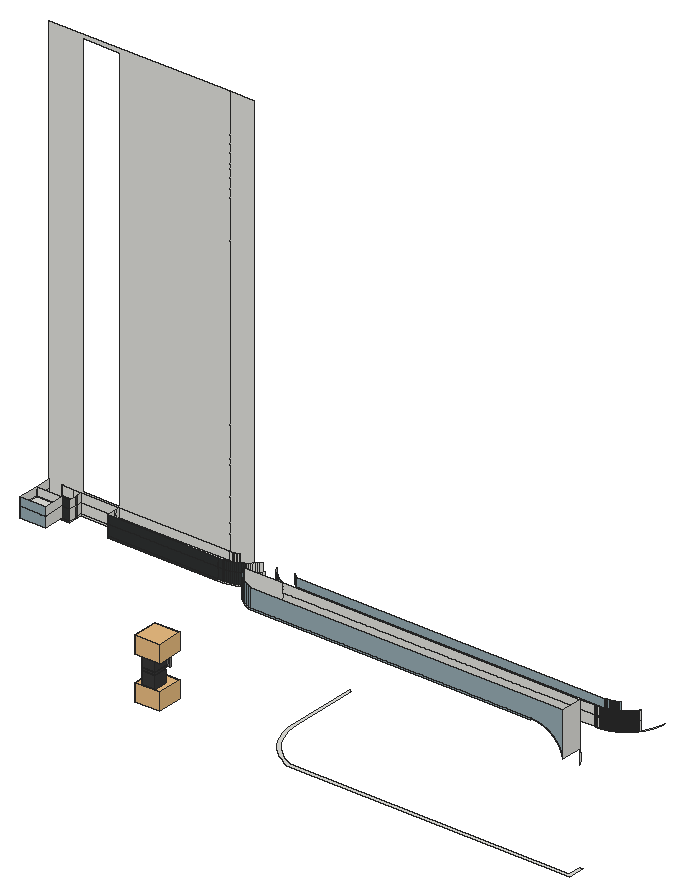
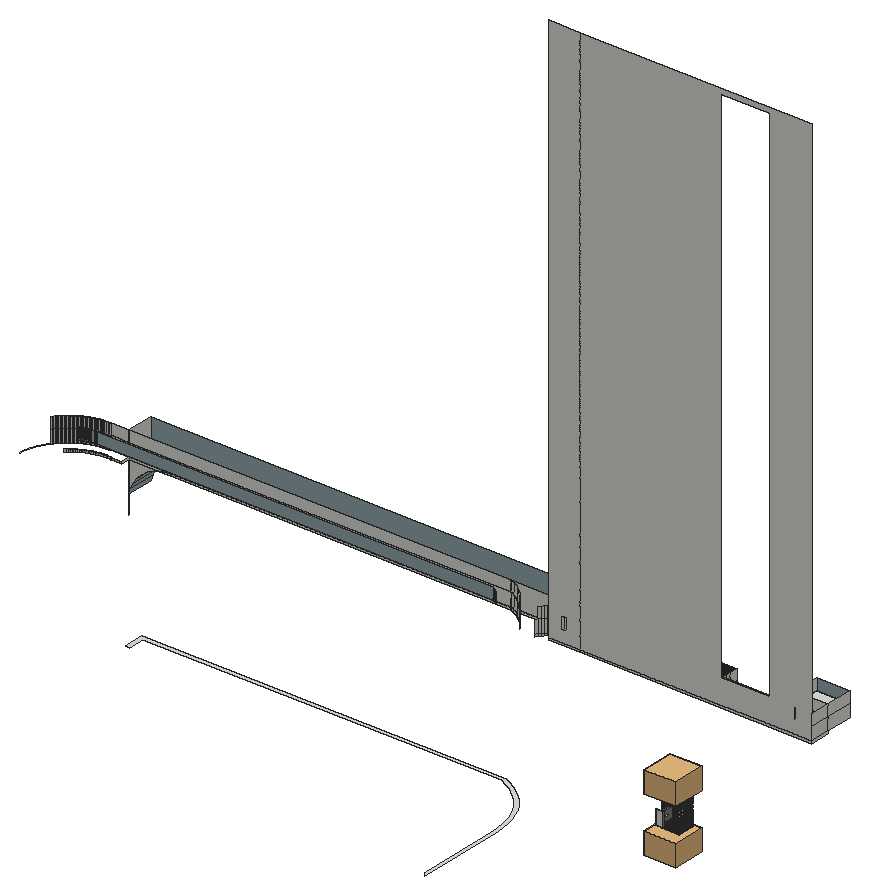
# SketchUp Ruby script. Lengths in inches.
U = 1.inch
M = Sketchup.active_model
def pt(a) = Geom::Point3d.new(a.map { |v| v * U })
def face(e, loops, mat)
  f = e.add_face(loops[0].map { |a| pt(a) })
  loops[1..].each { |l| e.add_face(l.map { |a| pt(a) }).erase! }
  f.material = f.back_material = mat if mat
  f
end
# faces: each face lists its corners as indices into pts; further lists are holes
def faces(e, pts, list, mat = nil) = list.each { |f| face(e, (f[0].is_a?(Array) ? f : [f]).map { |l| l.map { |i| pts[i] } }, mat) }
# xy, xz, yz: faces in a plane at the given z, y or x. An outline is a flat list of corners, or four numbers for a rectangle; further outlines are holes
def ring(l) = l.size == 4 ? [[l[0], l[1]], [l[2], l[1]], [l[2], l[3]], [l[0], l[3]]] : l.each_slice(2).to_a
def flat(e, list, mat, &to3) = list.each { |f| face(e, (f[0].is_a?(Array) ? f : [f]).map { |l| ring(l).map { |u, v| to3.(u, v) } }, mat) }
def xy(e, z, list, mat = nil) = flat(e, list, mat) { |x, y| [x, y, z] }
def xz(e, y, list, mat = nil) = flat(e, list, mat) { |x, z| [x, y, z] }
def yz(e, x, list, mat = nil) = flat(e, list, mat) { |y, z| [x, y, z] }
def lines(e, pts, list) = list.each { |a, b| e.add_line(pt(pts[a]), pt(pts[b])) }
# prism: a flat outline (further loops are holes) pulled along v
def prism(e, loops, v, mat = nil)
  f = face(e, loops, mat); d = Geom::Vector3d.new(v.map { |x| x * U })
  f.pushpull(f.normal.samedirection?(d) ? d.length : -d.length)
end
def box(e, o, s, mat = nil) = prism(e, [[o, [o[0] + s[0], o[1], o[2]], [o[0] + s[0], o[1] + s[1], o[2]], [o[0], o[1] + s[1], o[2]]]], [0, 0, s[2]], mat)
def at(x, y, z, deg = 0) = Geom::Transformation.translation(pt([x, y, z])) * Geom::Transformation.rotation(ORIGIN, Z_AXIS, deg.degrees)
def axes(o, x, y, z) = Geom::Transformation.new([*x, 0, *y, 0, *z, 0, *pt(o).to_a, 1])
def part(name) = M.definitions.add(name)
# library, detail: a bought-in or finely detailed component or shape, given as its bounding box
def library(name, o, s) = part(name).tap { |d| box(d.entities, o, s) }
def detail(e, o, s) = box(e.add_group.entities, o, s)
def put(e, d, t, mat = nil) = e.add_instance(d, t).tap { |i| i.material = mat if mat }
def group(e, t, mat = nil) = e.add_group.tap { |g| g.transformation = t; g.material = mat if mat }.entities
root = M.entities
M.materials.add("11.free-metal-textures").color = [58, 58, 58]
M.materials.add("Generic").color = [150, 171, 178]
M.materials.add("Generic\#1").color = [47, 50, 50]
M.materials.add("Glass Thin Clear 001").color = [252, 250, 250]
M.materials["Glass Thin Clear 001"].alpha = 0.1
M.materials.add("[0111_SlateGray]").color = [112, 128, 144]
M.materials.add("[0117_GhostWhite]").color = [248, 248, 255]
M.materials.add("images").color = [124, 124, 124]
c1 = library("Spot Light",[-7.3,-7.3,-9.9375],[14.6,14.6,9.9375])
c2 = part("Group0\#1")
p = [[-17.97,0.98,0],[-6.48,-16.79,0],[0,0,38],[13.97,-11.35,0],[15.11,9.78,0],[-4.625,17.4,0]]
faces(c2.entities,p,[[0,1,2],[1,3,2],[3,4,2],[5,0,2],[4,5,2]])
c3 = part("wall light")
g1 = group(c3.entities,at(188.14,62.59,-1.03))
xy(g1,0.24,[[[0,0,7.875,7.875],[0.49,0.49,7.38,7.38]]],"images")
xy(g1,1.03,[[[0.49,0.49,7.38,7.38],[0.73,0.73,7.14,7.14]]],"[0111_SlateGray]")
xy(g1,2.21,[[0.73,0.73,7.14,7.14]],"[0117_GhostWhite]")
xy(g1,5.75,[[2.36,13.78,5.51,14.17]],"images")
xy(g1,6.74,[[3.35,7.875,4.52,13.78]],"images")
xy(g1,7.72,[[0,0,7.875,0,7.875,7.875,7.38,7.875,7.38,0.49,0.49,0.49,0.49,7.875,0,7.875],[0.49,7.38,7.38,7.875]])
xy(g1,8.5,[[3.35,9.63,4.52,12.02]])
xy(g1,8.51,[[0,0,0,7.875,0.49,7.875,0.49,0.49,7.38,0.49,7.38,7.875,7.875,7.875,7.875,0]])
xy(g1,9.29,[[0,0,7.875,0,7.875,7.875,7.38,7.875,7.38,0.49,0.49,0.49,0.49,7.875,0,7.875]])
xy(g1,9.3,[[3.35,9.63,4.52,12.02]])
xy(g1,10.08,[[0,0,7.875,0,7.875,7.875,7.38,7.875,7.38,0.49,0,0.49],[0,0.49,0.49,7.875],[0.49,7.38,7.38,7.875]])
xy(g1,11.06,[[3.35,7.875,4.52,13.78]],"images")
xy(g1,12.05,[[2.36,13.78,5.51,14.17]],"images")
xy(g1,15.59,[[0.73,0.73,7.14,7.14]],"[0117_GhostWhite]")
xy(g1,16.77,[[[0.49,0.49,7.38,7.38],[0.73,0.73,7.14,7.14]]],"[0111_SlateGray]")
xy(g1,17.5625,[[[0,0,7.875,7.875],[0.49,0.49,7.38,7.38]]],"images")
xz(g1,0,[[0,0.24,7.875,7.72],[0,8.51,7.875,9.29],[0,10.08,7.875,17.5625]],"11.free-metal-textures")
xz(g1,0.49,[[0.49,8.51,7.38,8.9],[0.49,8.9,7.38,9.29]])
xz(g1,0.49,[[0.49,0.24,7.38,1.03],[0.49,16.77,7.38,17.5625]],"[0111_SlateGray]")
xz(g1,0.49,[[0.49,7.72,7.38,8.51],[0.49,9.29,7.38,10.08]],"[0117_GhostWhite]")
xz(g1,0.73,[[0.73,1.03,7.14,2.21],[0.73,2.21,7.14,15.59],[0.73,15.59,7.14,16.77]],"[0111_SlateGray]")
xz(g1,7.14,[[0.73,1.03,7.14,2.21],[0.73,2.21,7.14,15.59],[0.73,15.59,7.14,16.77]],"[0111_SlateGray]")
xz(g1,7.38,[[0.49,0.24,7.38,1.03],[0.49,16.77,7.38,17.5625]],"[0111_SlateGray]")
xz(g1,7.875,[[3.35,6.74,4.52,7.72],[3.35,7.72,3.9375,10.08],[3.9375,7.72,4.52,10.08],[3.35,10.08,4.52,11.06]])
xz(g1,7.875,[[0,0.24,0,7.72,3.35,7.72,3.35,6.74,4.52,6.74,4.52,7.72,7.875,7.72,7.875,0.24],[0.49,7.72,0.49,8.51,0,8.51,0,9.29,0.49,9.29,0.49,10.08,3.35,10.08,3.35,7.72],[4.52,7.72,4.52,10.08,7.38,10.08,7.38,9.29,7.875,9.29,7.875,8.51,7.38,8.51,7.38,7.72],[0,10.08,0,17.5625,7.875,17.5625,7.875,10.08,4.52,10.08,4.52,11.06,3.35,11.06,3.35,10.08]],"11.free-metal-textures")
xz(g1,9.63,[[3.35,8.5,4.52,9.3]])
xz(g1,12.02,[[3.35,8.5,4.52,9.3]])
xz(g1,13.78,[[2.36,5.75,4.52,5.75,4.52,6.74,3.35,6.74,3.35,11.06,4.52,11.06,4.52,5.75,5.51,5.75,5.51,12.05,2.36,12.05]],"images")
xz(g1,14.17,[[2.36,5.75,5.51,12.05]])
yz(g1,0,[[0,0.24,7.875,7.72],[0,8.51,7.875,9.29],[0,10.08,7.875,17.5625]],"11.free-metal-textures")
yz(g1,0.49,[[0.49,8.51,7.38,8.9]])
yz(g1,0.49,[[0.49,0.24,7.38,1.03],[0.49,16.77,7.38,17.5625]],"[0111_SlateGray]")
yz(g1,0.49,[[0.49,7.72,7.875,8.51],[0.49,9.29,7.875,10.08]],"[0117_GhostWhite]")
yz(g1,0.73,[[0.73,1.03,7.14,2.21],[0.73,2.21,7.14,15.59],[0.73,15.59,7.14,16.77]],"[0111_SlateGray]")
yz(g1,2.36,[[13.78,5.75,14.17,12.05]],"images")
yz(g1,3.35,[[[7.875,6.74,13.78,11.06],[9.63,8.5,12.02,9.3]]],"images")
yz(g1,4.52,[[[7.875,6.74,13.78,11.06],[9.63,8.5,12.02,9.3]]],"images")
yz(g1,5.51,[[13.78,5.75,14.17,12.05]],"images")
yz(g1,7.14,[[0.73,1.03,7.14,2.21],[0.73,2.21,7.14,15.59],[0.73,15.59,7.14,16.77]],"[0111_SlateGray]")
yz(g1,7.38,[[0.49,8.51,7.38,8.9]])
yz(g1,7.38,[[0.49,0.24,7.38,1.03],[0.49,16.77,7.38,17.5625]],"[0111_SlateGray]")
yz(g1,7.38,[[0.49,7.72,7.875,8.51],[0.49,9.29,7.875,10.08]],"[0117_GhostWhite]")
yz(g1,7.875,[[0,0.24,7.875,7.72],[0,8.51,7.875,9.29],[0,10.08,7.875,17.5625]],"11.free-metal-textures")
p = [[7.38,7.38,8.9],[0.49,7.38,8.9],[4.52,7.875,6.54],[4.52,7.875,6.74],[4.52,13.78,5.5625],[4.52,13.78,5.75]]
lines(g1,p,[[0,1],[2,3],[4,5]])
put(g1,c2,axes([3.74,4.28,0],[0.1617,0,0],[0,0.1617,0],[0,0,0.1617]))
put(g1,c2,axes([4.15,3.625,18],[-0.1617,0,0],[0,0.1617,0],[0,0,-0.1617]))
xy(root,168.5625,[[164.303,33.128,330.023,33.128,330.023,42.441,328.27,42.441,328.27,34.881,164.664,34.881,162.347,35.879,159.469,37.48,156.769,39.364,154.272,41.512,152.005,43.9,149.992,46.506,148.252,49.301,146.803,52.258,145.661,55.347,144.836,58.535,144.338,61.79,144.165,65.204,144.165,104.598,142.412,106.351,142.412,65.159,142.591,61.612,143.116,58.182,143.985,54.822,145.189,51.567,146.716,48.45,148.55,45.504,150.673,42.758,153.062,40.24,155.693,37.977,158.539,35.992,161.572,34.304]])
xy(root,245,[[145.638,29.933,143.73,30.488,141.889,31.231,140.131,32.157,138.476,33.255,136.939,34.513,135.537,35.921,134.284,37.462,133.193,39.122,132.274,40.883,131.803,42.0625,309.912,42.0625,309.912,29.933]],"Generic")
xy(root,246,[[10.218,29.933,25.218,42.0625],[145.638,29.933,309.912,29.933,309.912,42.0625,131.803,42.0625,132.274,40.883,133.193,39.122,134.284,37.462,135.537,35.921,136.939,34.513,138.476,33.255,140.131,32.157,141.889,31.231,143.73,30.488],[119.415,42.0625,120.438,42.148,121.455,42.289,122.463,42.485,123.459,42.737,124.439,43.042,125.401,43.4,126.342,43.81,127.26,44.271,128.151,44.781,129.013,45.339,129.843,45.943,130.639,46.592,129.741,45.931,128.812,45.317,127.853,44.749,126.867,44.231,125.856,43.763,124.822,43.346,123.769,42.981,122.699,42.67,121.615,42.412,120.52,42.21],[131.803,42.0625,131.651,42.423,131.509,42.788,131.377,43.156,131.254,43.528,131.142,43.903,131.039,44.28,130.947,44.661,130.865,45.043,130.793,45.428,130.731,45.814,130.68,46.202,130.639,46.592,130.991,44.637,131.538,42.727],[337.222,42.0625,337.846,42.071,338.474,42.095,339.101,42.136,339.638,42.186],
  [339.638,42.186,339.726,42.194,340.35,42.268,340.972,42.358,341.591,42.464,342.207,42.587,342.82,42.726,343.429,42.88,344.034,43.051,344.634,43.237,345.229,43.439,345.818,43.657,346.402,43.889,346.979,44.137,347.55,44.4,348.113,44.678,348.669,44.971,349.218,45.278,349.758,45.599,350.289,45.934,350.811,46.283,351.324,46.646,351.828,47.022,352.321,47.411,352.804,47.813,353.277,48.227,353.738,48.654,354.188,49.092,354.627,49.542,355.053,50.003,355.467,50.476,355.869,50.959,356.258,51.452,356.634,51.956,356.997,52.469,357.346,52.991,357.681,53.523,358.002,54.0625,358.309,54.611,358.602,55.167,358.88,55.73,359.143,56.301,359.391,56.878,359.624,57.462,359.841,58.051,360.043,58.646,360.229,59.246,360.4,59.851,360.554,60.46,360.693,61.073,360.816,61.689,360.922,62.308,361.012,62.93,361.086,63.554,361.094,63.642,361.086,63.17,361.031,62.701,360.967,62.234,360.893,61.768,360.81,61.304,360.718,60.841,360.617,60.381,360.506,59.922,360.387,59.466,360.258,59.012,360.12,58.561,359.973,58.113,359.818,57.668,359.653,57.226,359.48,56.787,359.298,56.352,359.107,55.921,358.908,55.494,358.701,55.07,358.484,54.651,358.26,54.236,358.027,53.826,357.787,53.421,357.538,53.02,357.281,52.624,357.016,52.234,356.744,51.849,356.464,51.47,356.176,51.096,355.881,50.728,355.579,50.366,355.27,50.01,354.953,49.66,354.63,49.317,354.3,48.98,353.963,48.65,353.62,48.327,353.27,48.01,352.914,47.701,352.552,47.399,352.184,47.104,351.81,46.816,351.431,46.536,351.046,46.264,350.656,45.999,350.26,45.742,349.859,45.494,349.454,45.253,349.044,45.02,348.629,44.796,348.21,44.58,347.786,44.372,347.359,44.173,346.928,43.982,346.493,43.8,346.054,43.627,345.612,43.462,345.167,43.307,344.719,43.16,344.268,43.022,343.814,42.893,343.358,42.774,342.899,42.663,342.439,42.562,341.976,42.47,341.512,42.387,341.046,42.313,340.579,42.249,340.111,42.194]])
xy(root,252,[[10.218,29.933,25.218,42.0625],[51.935,42.0625,51.935,50.129,118.879,50.129,119.252,50.179,119.415,50.209,119.415,42.0625],[119.415,42.0625,120.52,42.21,121.615,42.412,122.699,42.67,123.769,42.981,124.822,43.346,125.856,43.763,126.867,44.231,127.853,44.749,128.812,45.317,129.741,45.931,130.639,46.592,129.843,45.943,129.013,45.339,128.151,44.781,127.26,44.271,126.342,43.81,125.401,43.4,124.439,43.042,123.459,42.737,122.463,42.485,121.455,42.289,120.438,42.148]])
xz(root,29.933,[[328.648,231.068,328.648,257,145.638,257,145.638,246,309.912,246,312.78,245.785,315.583,245.145,318.259,244.093,320.749,242.655,322.996,240.861,324.951,238.751,326.569,236.374,327.814,233.783],[145.638,245,309.912,246],[10.218,246,25.218,252],[10.218,252,25.218,257]],"Generic")
xz(root,42.0625,[[328.648,222.472,328.648,231.068,328.659,231.034,329.084,228.19,329.081,225.315],[328.648,231.068,327.814,233.783,326.569,236.374,324.951,238.751,322.996,240.861,320.749,242.655,318.259,244.093,315.951,245,328.648,245],[10.218,245,25.218,246],[116.202,245,116.234,246],[116.234,245,119.415,246],
  [131.803,245,154.672,246],[154.672,245,309.912,246],[309.912,245,315.951,245,315.583,245.145,312.78,245.785,309.912,246],[315.951,245,315.583,245.145,312.78,245.785,309.912,246,328.648,246,328.648,245],[10.218,246,25.218,252],
  [116.202,246,116.234,252],[131.803,246,154.672,257],[154.672,246,328.648,252],[328.648,246,337.218,252],[337.218,246,337.222,252],
  [337.218,246,337.222,257],[10.218,252,25.218,257],[116.202,252,116.234,257],[154.672,252,328.648,257],[328.648,252,337.218,257],
  [337.218,252,337.222,257]])
xz(root,42.0625,[[25.218,245,29.81,246],[51.935,245,116.202,246],[25.218,246,29.81,252],[51.935,246,116.202,252],[116.234,246,119.415,252],
  [25.218,252,29.81,257],[51.935,252,116.202,257],[116.234,252,119.415,257]],"Generic\#1")
xz(root,46.0625,[[328.648,245,333.218,246]])
xz(root,50.129,[[29.81,245,51.935,246],[29.81,246,51.935,252],[18.284,252,25.218,257],[25.218,252,29.81,257],[29.81,252,51.935,257],
  [51.935,252,116.202,257],[116.202,252,118.879,257]])
xz(root,50.129,[[156.484,252,337.165,257]],"Generic")
xz(root,51.0625,[[10.218,245,116.202,246],[116.202,245,130.218,246],[[10.218,246,116.202,498],[29.81,257,51.935,495.654]],[116.202,246,130.218,498]])
yz(root,10.218,[[42.0625,245,51.0625,246],[29.933,246,42.0625,252],[42.0625,246,51.0625,252],[29.933,252,42.0625,257],[42.0625,252,51.0625,257]])
yz(root,18.284,[[50.129,252,51.0625,257]])
yz(root,25.218,[[29.933,246,42.0625,252],[29.933,252,42.0625,257]])
yz(root,29.81,[[42.0625,245,46.096,246],[47.721,245,50.129,246],[42.0625,246,46.096,252],[47.721,246,50.129,252],[42.0625,252,46.096,257],
  [47.721,252,50.129,257]])
yz(root,29.81,[[46.096,245,47.721,246],[46.096,246,47.721,252],[46.096,252,47.721,257]],"Glass Thin Clear 001")
yz(root,51.935,[[42.0625,245,46.096,246],[46.096,245,47.721,246],[47.721,245,50.129,246],[42.0625,246,46.096,252],[46.096,246,47.721,252],
  [47.721,246,50.129,252],[42.0625,252,46.096,257],[46.096,252,47.721,257],[47.721,252,50.129,257]])
yz(root,309.912,[[29.933,245,42.0625,246]])
yz(root,328.648,[[29.933,231.068,42.0625,257],[42.0625,245,46.0625,246]])
p = [[327.814,42.0625,233.783],[328.648,42.0625,231.068],[328.648,29.933,231.068],[327.814,29.933,233.783],[326.569,42.0625,236.374],[326.569,29.933,236.374],
  [324.951,42.0625,238.751],[324.951,29.933,238.751],[322.996,42.0625,240.861],[322.996,29.933,240.861],[320.749,42.0625,242.655],[320.749,29.933,242.655],
  [318.259,42.0625,244.093],[318.259,29.933,244.093],[315.951,42.0625,245],[315.583,29.933,245.145],[315.583,42.0625,245.145],[145.638,29.933,246],
  [143.73,30.488,246],[143.73,30.488,245],[145.638,29.933,245],[141.889,31.231,246],[141.889,31.231,245],[140.131,32.157,246],
  [140.131,32.157,245],[138.476,33.255,246],[138.476,33.255,245],[136.939,34.513,246],[136.939,34.513,245],[135.537,35.921,246],
  [135.537,35.921,245],[134.284,37.462,246],[134.284,37.462,245],[133.193,39.122,246],[133.193,39.122,245],[132.274,40.883,246],
  [132.274,40.883,245],[131.803,42.0625,246],[131.803,42.0625,245],[120.52,42.21,246],[119.415,42.0625,246],[119.415,42.0625,245],
  [120.52,42.21,245],[131.538,42.727,246],[131.538,42.727,245],[152.46,43.109,245],[152.46,43.109,246],[154.672,42.0625,246],
  [154.672,42.0625,245],[121.615,42.412,246],[121.615,42.412,245],[122.699,42.67,246],[122.699,42.67,245],[123.769,42.981,246],
  [123.769,42.981,245],[130.991,44.637,246],[130.991,44.637,245],[124.822,43.346,246],[124.822,43.346,245],[150.36,44.367,245],
  [150.36,44.367,246],[125.856,43.763,246],[125.856,43.763,245],[126.867,44.231,246],[126.867,44.231,245],[127.853,44.749,246],
  [127.853,44.749,245],[148.394,45.823,245],[148.394,45.823,246],[130.639,46.592,246],[130.639,46.592,245],[128.812,45.317,246],
  [128.812,45.317,245],[129.741,45.931,246],[129.741,45.931,245],[146.578,47.464,245],[146.578,47.464,246],[333.218,46.0625,246],
  [333.862,46.006,246],[333.862,46.006,245],[333.218,46.0625,245],[334.509,45.969,246],[334.509,45.969,245],[335.156,45.951,246],
  [335.156,45.951,245],[335.803,45.953,246],[335.803,45.953,245],[336.45,45.973,246],[336.45,45.973,245],[337.096,46.012,246],
  [337.096,46.012,245],[337.741,46.071,246],[337.741,46.071,245],[338.383,46.148,246],[338.383,46.148,245],[339.023,46.245,246],
  [339.023,46.245,245],[339.66,46.36,246],[339.66,46.36,245],[340.293,46.495,246],[340.293,46.495,245],[340.922,46.647,246],
  [340.922,46.647,245],[131.502,47.296,246],[131.502,47.296,245],[341.546,46.819,246],[341.546,46.819,245],[342.165,47.009,246],
  [342.165,47.009,245],[342.778,47.216,246],[342.778,47.216,245],[343.385,47.442,246],[343.385,47.442,245],[132.329,48.043,246],
  [132.329,48.043,245],[343.984,47.686,246],[343.984,47.686,245],[144.932,49.275,245],[144.932,49.275,246],[344.576,47.948,246],
  [344.576,47.948,245],[345.161,48.227,246],[345.161,48.227,245],[133.117,48.831,246],[133.117,48.831,245],[345.736,48.523,246],
  [345.736,48.523,245],[346.303,48.835,246],[346.303,48.835,245],[133.865,49.657,246],[133.865,49.657,245],[346.86,49.165,246],
  [346.86,49.165,245],[347.407,49.511,246],[347.407,49.511,245],[143.47,51.238,245],[143.47,51.238,246],[347.944,49.873,246],
  [347.944,49.873,245],[134.57,50.52,246],[134.57,50.52,245],[348.47,50.25,246],[348.47,50.25,245],[348.984,50.643,246],
  [348.984,50.643,245],[135.231,51.417,246],[135.231,51.417,245],[349.486,51.051,246],[349.486,51.051,245],[349.977,51.474,246],
  [349.977,51.474,245],[135.846,52.346,246],[135.846,52.346,245],[350.454,51.911,246],[350.454,51.911,245],[312.78,42.0625,245.785],
  [312.78,29.933,245.785],[309.912,42.0625,246],[309.912,29.933,246],[145.638,29.933,257],[143.73,30.488,257],[141.889,31.231,257],
  [140.131,32.157,257],[138.476,33.255,257],[136.939,34.513,257],[135.537,35.921,257],[134.284,37.462,257],[133.193,39.122,257],
  [132.274,40.883,257],[131.803,42.0625,257],[119.415,42.0625,252],[120.438,42.148,252],[120.438,42.148,246],[120.52,42.21,252],
  [121.455,42.289,252],[121.455,42.289,246],[131.538,42.727,257],[131.651,42.423,257],[131.651,42.423,246],[152.46,43.109,252],
  [154.672,42.0625,252],[337.846,42.071,252],[337.222,42.0625,252],[337.222,42.0625,246],[337.846,42.071,246],[338.474,42.095,246],
  [338.474,42.095,252],[339.101,42.136,246],[339.101,42.136,252],[339.638,42.186,246],[339.638,42.186,252],[121.615,42.412,252],
  [340.111,42.194,246],[340.111,42.194,252],[340.579,42.249,246],[340.579,42.249,252],[341.046,42.313,246],[341.046,42.313,252],
  [122.463,42.485,252],[122.463,42.485,246],[341.512,42.387,246],[341.512,42.387,252],[122.699,42.67,252],[131.509,42.788,257],
  [131.509,42.788,246],[341.976,42.47,246],[341.976,42.47,252],[123.459,42.737,252],[123.459,42.737,246],[342.439,42.562,246],
  [342.439,42.562,252],[342.899,42.663,246],[342.899,42.663,252],[123.769,42.981,252],[124.439,43.042,252],[124.439,43.042,246],
  [130.991,44.637,257],[343.358,42.774,246],[343.358,42.774,252],[131.377,43.156,257],[131.377,43.156,246],[343.814,42.893,246],
  [343.814,42.893,252],[344.268,43.022,246],[344.268,43.022,252],[124.822,43.346,252],[125.401,43.4,252],[125.401,43.4,246],
  [344.719,43.16,246],[344.719,43.16,252],[150.36,44.367,252],[131.254,43.528,257],[131.254,43.528,246],[345.167,43.307,246],
  [345.167,43.307,252],[125.856,43.763,252],[345.612,43.462,246],[345.612,43.462,252],[126.342,43.81,252],[126.342,43.81,246],
  [131.142,43.903,257],[131.142,43.903,246],[346.054,43.627,246],[346.054,43.627,252],[346.493,43.8,246],[346.493,43.8,252],
  [126.867,44.231,252],[127.26,44.271,252],[127.26,44.271,246],[346.928,43.982,246],[346.928,43.982,252],[131.039,44.28,257],
  [131.039,44.28,246],[347.359,44.173,246],[347.359,44.173,252],[127.853,44.749,252],[347.786,44.372,246],[347.786,44.372,252],
  [128.151,44.781,252],[128.151,44.781,246],[130.947,44.661,257],[130.947,44.661,246],[148.394,45.823,252],[348.21,44.58,246],
  [348.21,44.58,252],[130.639,46.592,257],[130.639,46.592,252],[348.629,44.796,246],[348.629,44.796,252],[128.812,45.317,252],
  [130.865,45.043,257],[130.865,45.043,246],[129.013,45.339,252],[129.013,45.339,246],[349.044,45.02,246],[349.044,45.02,252],
  [130.793,45.428,257],[130.793,45.428,246],[349.454,45.253,246],[349.454,45.253,252],[129.741,45.931,252],[129.843,45.943,252],
  [129.843,45.943,246],[349.859,45.494,246],[349.859,45.494,252],[130.731,45.814,257],[130.731,45.814,246],[350.26,45.742,246],
  [350.26,45.742,252],[350.656,45.999,246],[350.656,45.999,252],[130.68,46.202,257],[130.68,46.202,246],[146.578,47.464,252],
  [351.046,46.264,246],[351.046,46.264,252],[351.431,46.536,246],[351.431,46.536,252],[351.81,46.816,246],[351.81,46.816,252],
  [131.502,47.296,252],[352.184,47.104,246],[352.184,47.104,252],[352.552,47.399,246],[352.552,47.399,252],[132.329,48.043,252],
  [352.914,47.701,246],[352.914,47.701,252],[144.932,49.275,252],[353.27,48.01,246],[353.27,48.01,252],[133.117,48.831,252],
  [353.62,48.327,246],[353.62,48.327,252],[353.963,48.65,246],[353.963,48.65,252],[354.3,48.98,246],[354.3,48.98,252],
  [133.865,49.657,252],[354.63,49.317,246],[354.63,49.317,252],[143.47,51.238,252],[354.953,49.66,246],[354.953,49.66,252],
  [134.57,50.52,252],[355.27,50.01,246],[355.27,50.01,252],[355.579,50.366,246],[355.579,50.366,252],[355.881,50.728,246],
  [355.881,50.728,252],[135.231,51.417,252],[356.176,51.096,246],[356.176,51.096,252],[356.464,51.47,246],[356.464,51.47,252],
  [135.846,52.346,252],[356.744,51.849,246],[356.744,51.849,252],[120.438,42.148,257],[119.415,42.0625,257],[120.52,42.21,257],
  [121.455,42.289,257],[152.46,43.109,257],[154.672,42.0625,257],[337.846,42.071,257],[337.222,42.0625,257],[338.474,42.095,257],
  [339.101,42.136,257],[339.638,42.186,257],[121.615,42.412,257],[340.111,42.194,257],[340.579,42.249,257],[341.046,42.313,257],
  [122.463,42.485,257],[341.512,42.387,257],[122.699,42.67,257],[341.976,42.47,257],[123.459,42.737,257],[342.439,42.562,257],
  [342.899,42.663,257],[123.769,42.981,257],[124.439,43.042,257],[343.358,42.774,257],[343.814,42.893,257],[344.268,43.022,257],
  [124.822,43.346,257],[125.401,43.4,257],[344.719,43.16,257],[150.36,44.367,257],[345.167,43.307,257],[125.856,43.763,257],
  [345.612,43.462,257],[126.342,43.81,257],[346.054,43.627,257],[346.493,43.8,257],[126.867,44.231,257],[127.26,44.271,257],
  [346.928,43.982,257],[347.359,44.173,257],[127.853,44.749,257],[347.786,44.372,257],[128.151,44.781,257],[148.394,45.823,257],
  [348.21,44.58,257],[348.629,44.796,257],[128.812,45.317,257],[129.013,45.339,257],[349.044,45.02,257],[349.454,45.253,257],
  [129.741,45.931,257],[129.843,45.943,257],[349.859,45.494,257],[350.26,45.742,257],[350.656,45.999,257],[146.578,47.464,257],
  [351.046,46.264,257],[351.431,46.536,257],[351.81,46.816,257],[131.502,47.296,257],[352.184,47.104,257],[352.552,47.399,257],
  [132.329,48.043,257],[352.914,47.701,257],[144.932,49.275,257],[353.27,48.01,257],[133.117,48.831,257],[353.62,48.327,257],
  [353.963,48.65,257],[354.3,48.98,257],[133.865,49.657,257],[354.63,49.317,257],[143.47,51.238,257],[354.953,49.66,257],
  [134.57,50.52,257],[355.27,50.01,257],[355.579,50.366,257],[119.252,50.179,252],[118.879,50.129,252],[118.879,50.129,257],
  [119.252,50.179,257],[156.484,50.129,252],[156.266,50.232,252],[156.266,50.232,257],[156.484,50.129,257],[337.635,50.135,252],
  [337.165,50.129,252],[337.165,50.129,257],[337.635,50.135,257],[338.051,50.152,252],[338.051,50.152,257],[119.415,50.209,252],
  [119.415,50.209,257],[119.95,50.308,257],[119.95,50.308,252],[154.844,51.084,252],[154.844,51.084,257],[338.468,50.179,252],
  [338.468,50.179,257],[339.198,50.246,252],[339.198,50.246,257],[339.567,50.253,252],[339.567,50.253,257],[120.64,50.472,252],
  [120.64,50.472,257],[339.867,50.294,252],[339.867,50.294,257],[340.174,50.342,252],[340.174,50.342,257],[340.479,50.397,252],
  [340.479,50.397,257],[340.784,50.458,252],[340.784,50.458,257],[355.881,50.728,257],[121.321,50.67,252],[121.321,50.67,257],
  [135.231,51.417,257],[341.087,50.524,252],[341.087,50.524,257],[341.389,50.597,252],[341.389,50.597,257],[341.69,50.676,252],
  [341.69,50.676,257],[121.991,50.902,252],[121.991,50.902,257],[341.988,50.761,252],[341.988,50.761,257],[356.176,51.096,257],
  [342.286,50.851,252],[342.286,50.851,257],[122.649,51.167,252],[122.649,51.167,257],[342.581,50.948,252],[342.581,50.948,257],
  [342.874,51.05,252],[342.874,51.05,257],[154.672,51.212,252],[153.511,52.071,252],[153.511,52.071,257],[154.672,51.212,257],
  [343.165,51.159,252],[343.165,51.159,257],[356.464,51.47,257],[123.293,51.466,252],[123.293,51.466,257],[343.454,51.273,252],
  [343.454,51.273,257],[343.74,51.393,252],[343.74,51.393,257],[344.024,51.518,252],[344.024,51.518,257],[123.921,51.796,252],
  [123.921,51.796,257],[344.306,51.65,252],[344.306,51.65,257],[356.744,51.849,257],[344.585,51.786,252],[344.585,51.786,257],
  [344.861,51.929,252],[344.861,51.929,257]]
faces(root,p,[[0,1,2,3],[4,0,3,5],[6,4,5,7],[8,6,7,9],[10,8,9,11],[12,10,11,13],[14,12,13,15,16],[155,16,15,156],
  [157,155,156,158],[159,160,18,17],[160,161,21,18],[161,162,23,21],[162,163,25,23],[163,164,27,25],[164,165,29,27],[165,166,31,29],
  [166,167,33,31],[167,168,35,33],[168,169,37,35],[169,177,178,37],[177,203,204,178],[203,219,220,204],[219,231,232,220],[231,240,241,232],
  [240,251,252,241],[251,260,261,252],[260,270,271,261],[270,276,277,271],[276,285,286,277],[285,291,292,286],[265,266,69,292,291],[425,426,427,428],
  [429,425,428,430],[437,429,430,438],[439,437,438,440],[441,439,440,442],[445,441,442,446],[447,445,446,448],[449,447,448,450],[451,449,450,452],
  [457,451,452,458],[459,457,458,460],[461,459,460,462],[465,461,462,466],[468,465,466,469],[472,468,469,473],[474,472,473,475],[480,474,475,481],
  [485,480,481,486],[487,485,486,488],[489,487,488,490],[493,489,490,494],[496,493,494,497],[498,496,497,499]],"Generic")
faces(root,p,[[17,18,19,20],[18,21,22,19],[21,23,24,22],[23,25,26,24],[25,27,28,26],[27,29,30,28],[29,31,32,30],[31,33,34,32],
  [33,35,36,34],[35,37,38,36],[39,40,41,42],[38,37,43,44],[45,46,47,48],[49,39,42,50],[51,49,50,52],[53,51,52,54],
  [44,43,55,56],[57,53,54,58],[59,60,46,45],[61,57,58,62],[63,61,62,64],[65,63,64,66],[67,68,60,59],[56,55,69,70],
  [71,65,66,72],[73,71,72,74],[75,76,68,67],[69,73,74,70],[77,78,79,80],[78,81,82,79],[81,83,84,82],[83,85,86,84],
  [85,87,88,86],[87,89,90,88],[89,91,92,90],[91,93,94,92],[93,95,96,94],[95,97,98,96],[97,99,100,98],[99,101,102,100],
  [70,69,103,104],[101,105,106,102],[105,107,108,106],[107,109,110,108],[109,111,112,110],[104,103,113,114],[111,115,116,112],[117,118,76,75],
  [115,119,120,116],[119,121,122,120],[114,113,123,124],[121,125,126,122],[125,127,128,126],[124,123,129,130],[127,131,132,128],[131,133,134,132],
  [135,136,118,117],[133,137,138,134],[130,129,139,140],[137,141,142,138],[141,143,144,142],[140,139,145,146],[143,147,148,144],[147,149,150,148],
  [146,145,151,152],[149,153,154,150],[173,170,40,39],[43,37,169,176],[179,180,47,46],[181,182,183,184],[184,185,186,181],[185,187,188,186],
  [187,189,190,188],[191,173,39,49],[189,192,193,190],[192,194,195,193],[194,196,197,195],[196,200,201,197],[202,191,49,51],[200,205,206,201],
  [205,209,210,206],[209,211,212,210],[213,202,51,53],[176,216,55,43],[211,217,218,212],[217,221,222,218],[221,223,224,222],[225,213,53,57],
  [223,228,229,224],[230,179,46,60],[228,233,234,229],[235,225,57,61],[233,236,237,234],[236,242,243,237],[242,244,245,243],[246,235,61,63],
  [244,249,250,245],[249,253,254,250],[255,246,63,65],[253,256,257,254],[262,230,60,68],[256,263,264,257],[216,265,266,69,55],[263,267,268,264],
  [269,255,65,71],[267,274,275,268],[274,278,279,275],[280,269,71,73],[278,283,284,279],[283,287,288,284],[287,289,290,288],[293,262,68,76],
  [266,280,73,69],[289,294,295,290],[294,296,297,295],[296,298,299,297],[266,300,103,69],[298,301,302,299],[301,303,304,302],[300,305,113,103],
  [303,306,307,304],[308,293,76,118],[306,309,310,307],[305,311,123,113],[309,312,313,310],[312,314,315,313],[314,316,317,315],[311,318,129,123],
  [316,319,320,317],[321,308,118,136],[319,322,323,320],[318,324,139,129],[322,325,326,323],[325,327,328,326],[327,329,330,328],[324,331,145,139],
  [329,332,333,330],[332,334,335,333],[331,336,151,145],[334,337,338,335],[341,340,170,173],[180,179,343,344],[345,346,182,181],[181,186,347,345],
  [186,188,348,347],[188,190,349,348],[350,341,173,191],[190,193,351,349],[193,195,352,351],[195,197,353,352],[197,201,355,353],[356,350,191,202],
  [201,206,357,355],[206,210,359,357],[210,212,360,359],[361,356,202,213],[212,218,363,360],[218,222,364,363],[222,224,365,364],[366,361,213,225],
  [224,229,368,365],[179,230,369,343],[229,234,370,368],[371,366,225,235],[234,237,372,370],[237,243,374,372],[243,245,375,374],[376,371,235,246],
  [245,250,378,375],[250,254,379,378],[380,376,246,255],[254,257,381,379],[230,262,383,369],[257,264,384,381],[264,268,385,384],[386,380,255,269],
  [268,275,388,385],[275,279,389,388],[390,386,269,280],[279,284,392,389],[284,288,393,392],[288,290,394,393],[262,293,395,383],[265,390,280,266],
  [290,295,396,394],[295,297,397,396],[297,299,398,397],[300,266,265,399],[299,302,400,398],[302,304,401,400],[305,300,399,402],[304,307,403,401],
  [293,308,404,395],[307,310,405,403],[311,305,402,406],[310,313,407,405],[313,315,408,407],[315,317,409,408],[318,311,406,410],[317,320,411,409],
  [308,321,412,404],[320,323,413,411],[324,318,410,414],[323,326,415,413],[326,328,416,415],[417,418,419,420],[431,417,420,432,433,434],[443,434,433,444],
  [328,330,453,416],[454,443,444,455],[331,324,414,456],[463,454,455,464],[330,333,467,453],[470,463,464,471],[333,335,482,467],[483,470,471,484],
  [491,483,484,492],[335,338,495,482]])
faces(root,p,[[170,171,172,40],[171,174,175,172],[174,198,199,175],[198,207,208,199],[207,214,215,208],[214,226,227,215],[226,238,239,227],[238,247,248,239],
  [247,258,259,248],[258,272,273,259],[272,281,282,273],[281,266,69,282],[170,171,339,340],[171,174,342,339],[174,198,354,342],[198,207,358,354],
  [207,214,362,358],[214,226,367,362],[226,238,373,367],[238,247,377,373],[247,258,382,377],[258,272,387,382],[272,281,391,387],[281,266,265,391],
  [421,422,423,424],[422,435,436,423],[476,477,478,479,436,435]],"Generic\#1")
put(root,c1,at(81.74,41,180.36))
put(root,c1,axes([81.74,41,195.54],[1,0,0],[0,1,0],[0,0,-1]))
put(root,c3,at(-110.42,-27.91,180.47))
